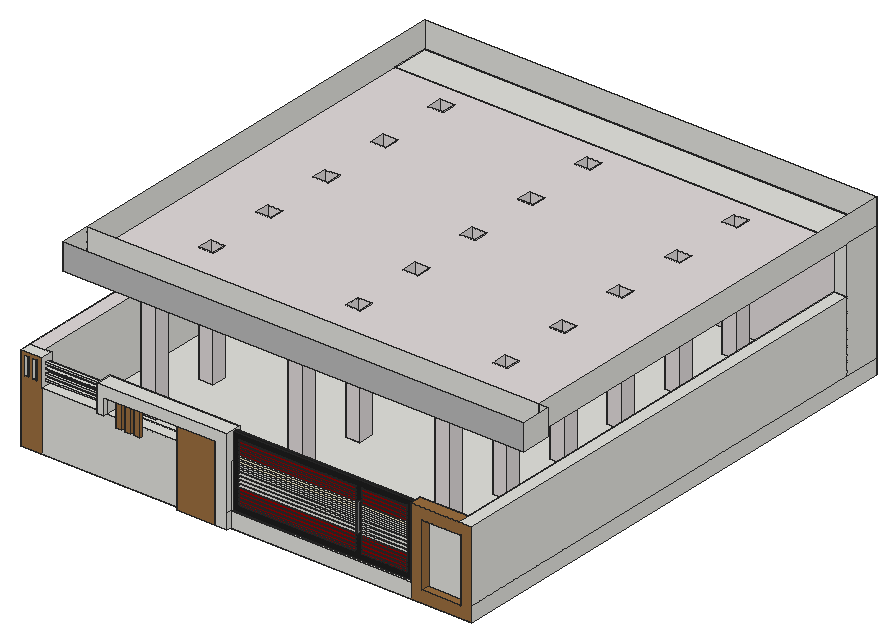
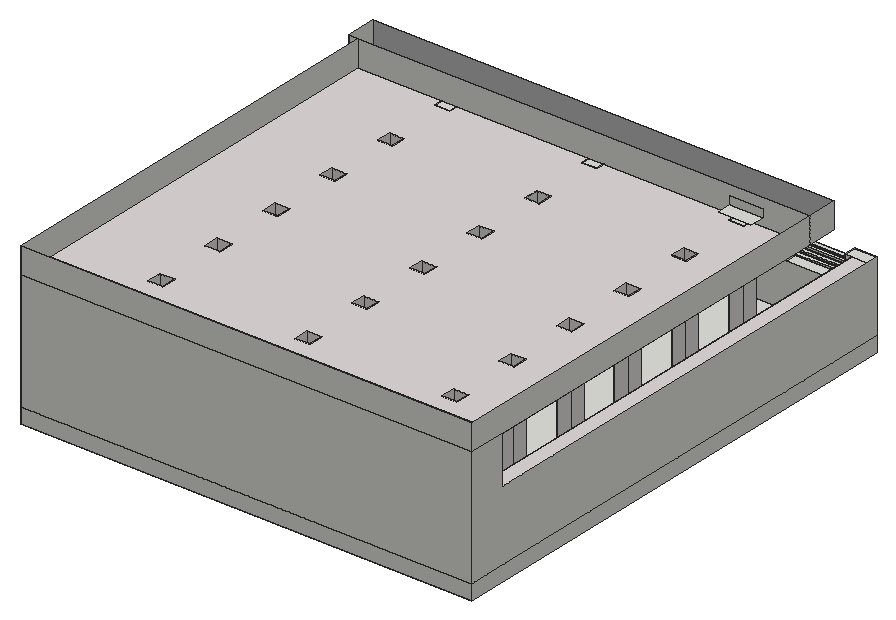
# SketchUp Ruby script. Lengths in inches.
U = 1.inch
M = Sketchup.active_model
def pt(a) = Geom::Point3d.new(a.map { |v| v * U })
def face(e, loops, mat)
  f = e.add_face(loops[0].map { |a| pt(a) })
  loops[1..].each { |l| e.add_face(l.map { |a| pt(a) }).erase! }
  f.material = f.back_material = mat if mat
  f
end
# faces: each face lists its corners as indices into pts; further lists are holes
def faces(e, pts, list, mat = nil) = list.each { |f| face(e, (f[0].is_a?(Array) ? f : [f]).map { |l| l.map { |i| pts[i] } }, mat) }
# xy, xz, yz: faces in a plane at the given z, y or x. An outline is a flat list of corners, or four numbers for a rectangle; further outlines are holes
def ring(l) = l.size == 4 ? [[l[0], l[1]], [l[2], l[1]], [l[2], l[3]], [l[0], l[3]]] : l.each_slice(2).to_a
def flat(e, list, mat, &to3) = list.each { |f| face(e, (f[0].is_a?(Array) ? f : [f]).map { |l| ring(l).map { |u, v| to3.(u, v) } }, mat) }
def xy(e, z, list, mat = nil) = flat(e, list, mat) { |x, y| [x, y, z] }
def xz(e, y, list, mat = nil) = flat(e, list, mat) { |x, z| [x, y, z] }
def yz(e, x, list, mat = nil) = flat(e, list, mat) { |y, z| [x, y, z] }
def lines(e, pts, list) = list.each { |a, b| e.add_line(pt(pts[a]), pt(pts[b])) }
# prism: a flat outline (further loops are holes) pulled along v
def prism(e, loops, v, mat = nil)
  f = face(e, loops, mat); d = Geom::Vector3d.new(v.map { |x| x * U })
  f.pushpull(f.normal.samedirection?(d) ? d.length : -d.length)
end
def box(e, o, s, mat = nil) = prism(e, [[o, [o[0] + s[0], o[1], o[2]], [o[0] + s[0], o[1] + s[1], o[2]], [o[0], o[1] + s[1], o[2]]]], [0, 0, s[2]], mat)
def at(x, y, z, deg = 0) = Geom::Transformation.translation(pt([x, y, z])) * Geom::Transformation.rotation(ORIGIN, Z_AXIS, deg.degrees)
def axes(o, x, y, z) = Geom::Transformation.new([*x, 0, *y, 0, *z, 0, *pt(o).to_a, 1])
def part(name) = M.definitions.add(name)
# library, detail: a bought-in or finely detailed component or shape, given as its bounding box
def library(name, o, s) = part(name).tap { |d| box(d.entities, o, s) }
def detail(e, o, s) = box(e.add_group.entities, o, s)
def put(e, d, t, mat = nil) = e.add_instance(d, t).tap { |i| i.material = mat if mat }
def group(e, t, mat = nil) = e.add_group.tap { |g| g.transformation = t; g.material = mat if mat }.entities
root = M.entities
M.materials.add("Generic").color = [155, 110, 63]
M.materials.add("Generic\#2").color = [186, 186, 186]
M.materials.add("Generic\#3").color = [224, 218, 218]
M.materials.add("[Color A07]").color = [153, 0, 0]
M.materials.add("[Color D01]").color = [255, 242, 204]
M.materials.add("[Color M04]").color = [142, 142, 142]
M.materials.add("[Color M08]").color = [30, 30, 30]
c1 = part("Group\#1")
xy(c1.entities,0,[[0,0,46.77,20.375]])
xz(c1.entities,0,[[0,0,46.77,11.0625]])
xy(root,-21.3125,[[275.43,0,329.375,6.375],[329.375,0,347.5625,6.375],[48.5,6.375,690.4375,724.5]])
xy(root,-5.23,[[619.21,6.375,674.35,18.4375]],"Generic")
xy(root,0.1875,[[[347.5625,6.375,603.125,6.375,603.125,23.0625,672,23.0625,672,672.375,69.875,672.375,69.875,23.0625,347.5625,23.0625],[132.71,115.57,153.71,136.82],[132.71,217.57,153.71,238.82],[132.71,319.57,153.71,340.82],[132.71,421.57,153.71,442.82],[132.71,523.57,153.71,544.82],[132.71,625.57,153.71,646.82],[341.56,625.57,362.56,646.82],[341.56,523.57,362.56,544.82],[341.56,421.57,362.56,442.82],[341.56,319.57,362.56,340.82],[341.56,217.57,362.56,238.82],[341.56,115.57,362.56,136.82],[550.4,625.57,571.4,646.82],[550.4,523.57,571.4,544.82],[550.4,421.57,571.4,442.82],[550.4,319.57,571.4,340.82],[550.4,217.57,571.4,238.82],[550.4,115.57,571.4,136.82]],[132.71,115.57,153.71,136.82],[341.56,115.57,362.56,136.82],[550.4,115.57,571.4,136.82],[132.71,217.57,153.71,238.82],
  [341.56,217.57,362.56,238.82],[550.4,217.57,571.4,238.82],[132.71,319.57,153.71,340.82],[341.56,319.57,362.56,340.82],[550.4,319.57,571.4,340.82],
  [132.71,421.57,153.71,442.82],[341.56,421.57,362.56,442.82],[550.4,421.57,571.4,442.82],[132.71,523.57,153.71,544.82],[341.56,523.57,362.56,544.82],
  [550.4,523.57,571.4,544.82],[132.71,625.57,153.71,646.82],[341.56,625.57,362.56,646.82],[550.4,625.57,571.4,646.82]])
xy(root,50.95,[[186.18,3.25,194.99,6.375],[199.43,3.25,208.24,6.375],[212.68,3.25,221.49,6.375]],"Generic")
xy(root,62.7,[[162.58,0,171.58,6.375],[79.4375,6.375,162.58,23.0625],[162.58,6.375,171.58,23.0625],[171.58,6.375,329.375,23.0625],[329.375,6.375,347.5625,23.0625]])
xy(root,69.64,[[54.75,6.375,60.37,9.625],[66.31,6.375,71.93,9.625]])
xy(root,70.21,[[79.4375,11.47,162.58,16.59],[162.58,11.47,164.83,16.59]])
xy(root,72.34,[[79.4375,11.47,162.58,16.59],[162.58,11.47,166.52,16.59]])
xy(root,77.4,[[79.4375,11.47,162.58,16.59],[162.58,11.47,166.52,16.59]])
xy(root,79.52,[[79.4375,11.47,162.58,16.59],[162.58,11.47,166.52,16.59]])
xy(root,84.59,[[79.4375,11.47,162.58,16.59],[162.58,11.47,166.52,16.59]])
xy(root,84.85,[[619.21,6.375,674.35,18.4375]],"Generic")
xy(root,85.75,[[171.58,0,275.43,6.375],[171.58,6.375,329.375,23.0625]])
xy(root,86.27,[[186.18,3.25,194.99,6.375],[199.43,3.25,208.24,6.375],[212.68,3.25,221.49,6.375]])
xy(root,86.71,[[79.4375,11.47,162.58,16.59],[162.58,11.47,166.52,16.59]])
xy(root,91.77,[[79.4375,11.47,162.58,16.59],[162.58,11.47,166.52,16.59]])
xy(root,93.9,[[79.4375,11.47,162.58,16.59],[162.58,11.47,164.83,16.59]])
xy(root,95.83,[[54.75,6.375,60.37,9.625],[66.31,6.375,71.93,9.625]])
xy(root,100.9375,[[162.58,0,347.5625,23.0625],[48.5,6.375,79.4375,23.0625],[672,6.375,690.4375,672.375]])
xy(root,100.9375,[[603.125,6.375,672,23.0625]],"Generic")
xy(root,100.9375,[[48.5,23.0625,69.875,672.375]],"Generic\#3")
xy(root,168,[[132.71,115.57,153.71,124.5],[341.56,115.57,362.56,124.5],[550.4,115.57,571.4,124.5],[132.71,124.5,153.71,136.82],[341.56,124.5,362.56,136.82],
  [550.4,124.5,571.4,136.82],[48.5,672.375,690.4375,724.5]])
xy(root,168,[[48.5,81.125,48.5,124.5,132.71,124.5,132.71,115.57,153.71,115.57,153.71,124.5,341.56,124.5,341.56,115.57,362.56,115.57,362.56,124.5,550.4,124.5,550.4,115.57,571.4,115.57,571.4,124.5,703.6875,124.5,703.6875,81.125]],"Generic\#2")
xy(root,168,[[[48.5,124.5,48.5,672.375,690.4375,672.375,690.4375,124.5,571.4,124.5,571.4,136.82,550.4,136.82,550.4,124.5,362.56,124.5,362.56,136.82,341.56,136.82,341.56,124.5,153.71,124.5,153.71,136.82,132.71,136.82,132.71,124.5],[132.71,625.57,153.71,646.82],[341.56,625.57,362.56,646.82],[550.4,625.57,571.4,646.82],[550.4,523.57,571.4,544.82],[341.56,523.57,362.56,544.82],[132.71,523.57,153.71,544.82],[341.56,421.57,362.56,442.82],[550.4,421.57,571.4,442.82],[132.71,421.57,153.71,442.82],[132.71,319.57,153.71,340.82],[341.56,319.57,362.56,340.82],[550.4,319.57,571.4,340.82],[550.4,217.57,571.4,238.82],[341.56,217.57,362.56,238.82],[132.71,217.57,153.71,238.82]]],"Generic\#3")
xz(root,0,[[329.375,-21.3125,347.5625,-21.3125,347.5625,100.9375,162.58,100.9375,162.58,62.7,171.58,62.7,171.58,85.75,329.375,85.75]])
xz(root,0,[[275.43,-21.3125,329.375,85.75]],"Generic")
xz(root,3.25,[[186.18,50.95,194.99,86.27],[199.43,50.95,208.24,86.27],[212.68,50.95,221.49,86.27]],"Generic")
xz(root,6.375,[[79.4375,-21.3125,275.43,-21.3125,275.43,62.7,221.49,62.7,221.49,50.95,212.68,50.95,212.68,62.7,208.24,62.7,208.24,50.95,199.43,50.95,199.43,62.7,194.99,62.7,194.99,50.95,186.18,50.95,186.18,62.7,79.4375,62.7],[275.43,-21.3125,329.375,62.7],[329.375,-21.3125,347.5625,62.7],[347.5625,-21.3125,603.125,0.1875],[186.18,50.95,194.99,62.7],
  [199.43,50.95,208.24,62.7],[212.68,50.95,221.49,62.7],[186.18,62.7,194.99,85.75],[199.43,62.7,208.24,85.75],[212.68,62.7,221.49,85.75],
  [275.43,62.7,329.375,85.75],[186.18,85.75,194.99,86.27],[199.43,85.75,208.24,86.27],[212.68,85.75,221.49,86.27]])
xz(root,6.375,[[[48.5,-21.3125,79.4375,100.9375],[54.75,69.64,60.37,95.83],[66.31,69.64,71.93,95.83]],[[603.125,-21.3125,690.4375,100.9375],[619.21,-5.23,674.35,84.85]]],"Generic")
xz(root,9.625,[[54.75,69.64,60.37,95.83],[66.31,69.64,71.93,95.83]])
xz(root,11.47,[[79.4375,70.21,162.58,72.34],[162.58,70.21,164.83,72.34],[164.83,72.34,166.52,77.4],[79.4375,77.4,162.58,79.52],[162.58,77.4,164.83,79.52],
  [164.83,79.52,166.52,84.59],[79.4375,84.59,162.58,86.71],[162.58,84.59,164.83,86.71],[164.83,86.71,166.52,91.77],[79.4375,91.77,162.58,93.9],
  [162.58,91.77,164.83,93.9]])
xz(root,16.59,[[79.4375,70.21,162.58,72.34],[162.58,70.21,164.83,72.34],[164.83,72.34,166.52,77.4],[79.4375,77.4,162.58,79.52],[162.58,77.4,164.83,79.52],
  [164.83,79.52,166.52,84.59],[79.4375,84.59,162.58,86.71],[162.58,84.59,164.83,86.71],[164.83,86.71,166.52,91.77],[79.4375,91.77,162.58,93.9],
  [162.58,91.77,164.83,93.9]])
xz(root,18.4375,[[619.21,-5.23,674.35,84.85]])
xz(root,23.0625,[[69.875,0.1875,347.5625,62.7],[603.125,0.1875,672,100.9375],[69.875,62.7,79.4375,100.9375],[162.58,62.7,162.58,100.9375,347.5625,100.9375,347.5625,62.7,329.375,62.7,329.375,85.75,171.58,85.75,171.58,62.7]])
xz(root,81.125,[[48.5,168,703.6875,204.9375]],"Generic\#2")
xz(root,115.57,[[132.71,0.1875,153.71,168],[341.56,0.1875,362.56,168],[550.4,0.1875,571.4,168]],"Generic\#3")
xz(root,124.5,[[48.5,168,690.4375,204.9375],[690.4375,168,703.6875,204.9375]])
xz(root,136.82,[[132.71,0.1875,153.71,168],[341.56,0.1875,362.56,168],[550.4,0.1875,571.4,168]],"Generic\#3")
xz(root,217.57,[[132.71,0.1875,153.71,168],[341.56,0.1875,362.56,168],[550.4,0.1875,571.4,168]],"Generic\#3")
xz(root,238.82,[[132.71,0.1875,153.71,168],[341.56,0.1875,362.56,168],[550.4,0.1875,571.4,168]],"Generic\#3")
xz(root,319.57,[[132.71,0.1875,153.71,168],[341.56,0.1875,362.56,168],[550.4,0.1875,571.4,168]],"Generic\#3")
xz(root,340.82,[[132.71,0.1875,153.71,168],[341.56,0.1875,362.56,168],[550.4,0.1875,571.4,168]],"Generic\#3")
xz(root,421.57,[[132.71,0.1875,153.71,168],[341.56,0.1875,362.56,168],[550.4,0.1875,571.4,168]],"Generic\#3")
xz(root,442.82,[[132.71,0.1875,153.71,168],[341.56,0.1875,362.56,168],[550.4,0.1875,571.4,168]],"Generic\#3")
xz(root,523.57,[[132.71,0.1875,153.71,168],[341.56,0.1875,362.56,168],[550.4,0.1875,571.4,168]],"Generic\#3")
xz(root,544.82,[[132.71,0.1875,153.71,168],[341.56,0.1875,362.56,168],[550.4,0.1875,571.4,168]],"Generic\#3")
xz(root,625.57,[[132.71,0.1875,153.71,168],[341.56,0.1875,362.56,168],[550.4,0.1875,571.4,168]],"Generic\#3")
xz(root,646.82,[[132.71,0.1875,153.71,168],[341.56,0.1875,362.56,168],[550.4,0.1875,571.4,168]],"Generic\#3")
xz(root,672.375,[[672,0.1875,690.4375,100.9375],[672,100.9375,690.4375,168]])
xz(root,672.375,[[69.875,0.1875,672,168],[48.5,100.9375,69.875,168]],"Generic\#3")
xz(root,724.5,[[48.5,-21.3125,690.4375,0.1875],[48.5,0.1875,690.4375,168],[48.5,168,690.4375,204.9375]])
yz(root,48.5,[[6.375,-21.3125,724.5,0.1875],[6.375,0.1875,6.375,100.9375,672.375,100.9375,672.375,168,724.5,168,724.5,0.1875],[81.125,168,124.5,204.9375],[124.5,168,724.5,204.9375]])
yz(root,54.75,[[6.375,69.64,9.625,95.83]])
yz(root,60.37,[[6.375,69.64,9.625,95.83]])
yz(root,66.31,[[6.375,69.64,9.625,95.83]])
yz(root,69.875,[[23.0625,0.1875,672.375,100.9375]])
yz(root,71.93,[[6.375,69.64,9.625,95.83]])
yz(root,79.4375,[[[6.375,62.7,23.0625,100.9375],[11.47,91.77,16.59,93.9],[11.47,84.59,16.59,86.71],[11.47,77.4,16.59,79.52],[11.47,70.21,16.59,72.34]]])
yz(root,132.71,[[115.57,0.1875,136.82,168],[217.57,0.1875,238.82,168],[319.57,0.1875,340.82,168],[421.57,0.1875,442.82,168],[523.57,0.1875,544.82,168],
  [625.57,0.1875,646.82,168]],"Generic\#3")
yz(root,153.71,[[115.57,0.1875,136.82,168],[217.57,0.1875,238.82,168],[319.57,0.1875,340.82,168],[421.57,0.1875,442.82,168],[523.57,0.1875,544.82,168],
  [625.57,0.1875,646.82,168]],"Generic\#3")
yz(root,162.58,[[[0,62.7,23.0625,100.9375],[11.47,70.21,16.59,72.34],[11.47,84.59,16.59,86.71],[11.47,77.4,16.59,79.52],[11.47,91.77,16.59,93.9]],[11.47,70.21,16.59,72.34],[11.47,77.4,16.59,79.52],[11.47,84.59,16.59,86.71],[11.47,91.77,16.59,93.9]])
yz(root,164.83,[[11.47,70.21,16.59,93.9]])
yz(root,166.52,[[11.47,72.34,16.59,77.4],[11.47,79.52,16.59,84.59],[11.47,86.71,16.59,91.77]])
yz(root,171.58,[[0,62.7,6.375,85.75],[6.375,62.7,23.0625,85.75]])
yz(root,186.18,[[3.25,50.95,6.375,86.27]],"Generic")
yz(root,194.99,[[3.25,50.95,6.375,86.27]],"Generic")
yz(root,199.43,[[3.25,50.95,6.375,86.27]],"Generic")
yz(root,208.24,[[3.25,50.95,6.375,86.27]],"Generic")
yz(root,212.68,[[3.25,50.95,6.375,86.27]],"Generic")
yz(root,221.49,[[3.25,50.95,6.375,86.27]],"Generic")
yz(root,275.43,[[0,-21.3125,6.375,85.75]],"Generic")
yz(root,329.375,[[0,-21.3125,6.375,85.75],[6.375,62.7,23.0625,85.75]])
yz(root,341.56,[[115.57,0.1875,136.82,168],[217.57,0.1875,238.82,168],[319.57,0.1875,340.82,168],[421.57,0.1875,442.82,168],[523.57,0.1875,544.82,168],
  [625.57,0.1875,646.82,168]],"Generic\#3")
yz(root,347.5625,[[0,-21.3125,6.375,0.1875],[0,0.1875,6.375,0.1875,6.375,62.7,23.0625,62.7,23.0625,100.9375,0,100.9375],[6.375,0.1875,23.0625,62.7]])
yz(root,362.56,[[115.57,0.1875,136.82,168],[217.57,0.1875,238.82,168],[319.57,0.1875,340.82,168],[421.57,0.1875,442.82,168],[523.57,0.1875,544.82,168],
  [625.57,0.1875,646.82,168]],"Generic\#3")
yz(root,550.4,[[115.57,0.1875,136.82,168],[217.57,0.1875,238.82,168],[319.57,0.1875,340.82,168],[421.57,0.1875,442.82,168],[523.57,0.1875,544.82,168],
  [625.57,0.1875,646.82,168]],"Generic\#3")
yz(root,571.4,[[115.57,0.1875,136.82,168],[217.57,0.1875,238.82,168],[319.57,0.1875,340.82,168],[421.57,0.1875,442.82,168],[523.57,0.1875,544.82,168],
  [625.57,0.1875,646.82,168]],"Generic\#3")
yz(root,603.125,[[6.375,0.1875,23.0625,100.9375]],"Generic")
yz(root,619.21,[[6.375,-5.23,18.4375,84.85]],"Generic")
yz(root,672,[[23.0625,0.1875,672.375,100.9375]])
yz(root,674.35,[[6.375,-5.23,18.4375,84.85]],"Generic")
yz(root,690.4375,[[6.375,-21.3125,724.5,0.1875],[6.375,0.1875,672.375,100.9375],[672.375,0.1875,724.5,168],[124.5,168,724.5,204.9375]])
yz(root,703.6875,[[81.125,168,124.5,204.9375]])
p = [[69.875,23.0625,0.1875],[69.875,6.375,0.1875],[162.58,13.96,70.93],[69.875,13.96,70.93],[162.58,13.96,78.18],[69.875,13.96,78.18],
  [162.58,13.96,85.43],[69.875,13.96,85.43],[162.58,13.96,92.68],[69.875,13.96,92.68]]
lines(root,p,[[0,1],[2,3],[4,5],[6,7],[8,9]])
g1 = group(root,at(347.5625,6.375,0.1875))
xy(g1,0,[[0,3.66,255.5625,8.66]],"[Color M08]")
xy(g1,10.64,[[8.11,3.66,175.29,8.66],[183.4,3.66,247.45,8.66]],"[Color A07]")
xy(g1,12.64,[[8.11,3.66,175.29,8.66],[183.4,3.66,247.45,8.66]],"[Color A07]")
xy(g1,15.64,[[8.11,3.66,175.29,8.66],[183.4,3.66,247.45,8.66]],"[Color A07]")
xy(g1,17.64,[[8.11,3.66,175.29,8.66],[183.4,3.66,247.45,8.66]],"[Color A07]")
xy(g1,20.64,[[8.11,3.66,175.29,8.66],[183.4,3.66,247.45,8.66]],"[Color A07]")
xy(g1,22.64,[[8.11,3.66,175.29,8.66],[183.4,3.66,247.45,8.66]],"[Color A07]")
xy(g1,25.64,[[8.11,3.66,175.29,8.66],[183.4,3.66,247.45,8.66]],"[Color A07]")
xy(g1,27.64,[[8.11,3.66,175.29,8.66],[183.4,3.66,247.45,8.66]],"[Color A07]")
xy(g1,30.64,[[8.11,3.66,175.29,8.66],[183.4,3.66,247.45,8.66]],"[Color A07]")
xy(g1,32.64,[[8.11,3.66,175.29,8.66],[183.4,3.66,247.45,8.66]])
xy(g1,35.04,[[178.11,0,180.64,3.66]])
xy(g1,35.64,[[8.11,3.66,175.29,8.66],[183.4,3.66,247.45,8.66]])
xy(g1,36.41,[[178.11,1.375,180.64,3.66]],"[Color M04]")
xy(g1,37.64,[[8.11,3.66,175.29,8.66],[183.4,3.66,247.45,8.66]])
xy(g1,40.64,[[8.11,3.66,175.29,8.66],[183.4,3.66,247.45,8.66]])
xy(g1,42.64,[[8.11,3.66,175.29,8.66],[183.4,3.66,247.45,8.66]])
xy(g1,45.64,[[8.11,3.66,175.29,8.66],[183.4,3.66,247.45,8.66]])
xy(g1,47.64,[[8.11,3.66,175.29,8.66],[183.4,3.66,247.45,8.66]])
xy(g1,50.64,[[8.11,3.66,175.29,8.66],[183.4,3.66,247.45,8.66]])
xy(g1,52.64,[[8.11,3.66,175.29,8.66],[183.4,3.66,247.45,8.66]])
xy(g1,55.64,[[8.11,3.66,175.29,8.66],[183.4,3.66,247.45,8.66]])
xy(g1,57.64,[[8.11,3.66,175.29,8.66],[183.4,3.66,247.45,8.66]])
xy(g1,60.64,[[8.11,3.66,175.29,8.66],[183.4,3.66,247.45,8.66]])
xy(g1,62.64,[[8.11,3.66,175.29,8.66],[183.4,3.66,247.45,8.66]])
xy(g1,65.64,[[8.11,3.66,175.29,8.66],[183.4,3.66,247.45,8.66]])
xy(g1,67.64,[[8.11,3.66,175.29,8.66],[183.4,3.66,247.45,8.66]])
xy(g1,70.64,[[8.11,3.66,175.29,8.66],[183.4,3.66,247.45,8.66]])
xy(g1,72.64,[[8.11,3.66,175.29,8.66],[183.4,3.66,247.45,8.66]],"[Color A07]")
xy(g1,73.21,[[178.11,1.375,180.64,3.66]],"[Color M04]")
xy(g1,74.59,[[178.11,0,180.64,3.66]])
xy(g1,75.64,[[8.11,3.66,175.29,8.66],[183.4,3.66,247.45,8.66]],"[Color A07]")
xy(g1,77.64,[[8.11,3.66,175.29,8.66],[183.4,3.66,247.45,8.66]],"[Color A07]")
xy(g1,80.64,[[8.11,3.66,175.29,8.66],[183.4,3.66,247.45,8.66]],"[Color A07]")
xy(g1,82.64,[[8.11,3.66,175.29,8.66],[183.4,3.66,247.45,8.66]],"[Color A07]")
xy(g1,85.64,[[8.11,3.66,175.29,8.66],[183.4,3.66,247.45,8.66]],"[Color A07]")
xy(g1,87.64,[[8.11,3.66,175.29,8.66],[183.4,3.66,247.45,8.66]],"[Color A07]")
xy(g1,90.64,[[8.11,3.66,175.29,8.66],[183.4,3.66,247.45,8.66]],"[Color A07]")
xy(g1,92.64,[[8.11,3.66,175.29,8.66],[183.4,3.66,247.45,8.66]])
xy(g1,100.75,[[0,3.66,255.5625,8.66]],"[Color M08]")
xz(g1,0,[[178.11,35.04,180.64,74.59]],"[Color M04]")
xz(g1,1.375,[[178.11,36.41,180.64,73.21]])
xz(g1,3.66,[[8.11,32.64,175.29,35.64],[183.4,32.64,247.45,35.64],[8.11,37.64,175.29,40.64],[183.4,37.64,247.45,40.64],[8.11,42.64,175.29,45.64],
  [183.4,42.64,247.45,45.64],[8.11,47.64,175.29,50.64],[183.4,47.64,247.45,50.64],[8.11,52.64,175.29,55.64],[183.4,52.64,247.45,55.64],
  [8.11,57.64,175.29,60.64],[183.4,57.64,247.45,60.64],[183.4,62.64,247.45,65.64],[178.11,73.21,180.64,74.59]])
xz(g1,3.66,[[8.11,8.11,175.29,10.64],[183.4,8.11,247.45,10.64],[8.11,12.64,175.29,15.64],[183.4,12.64,247.45,15.64],[8.11,17.64,175.29,20.64],
  [183.4,17.64,247.45,20.64],[8.11,22.64,175.29,25.64],[183.4,22.64,247.45,25.64],[8.11,27.64,175.29,30.64],[183.4,27.64,247.45,30.64],
  [8.11,72.64,175.29,75.64],[183.4,72.64,247.45,75.64],[8.11,77.64,175.29,80.64],[183.4,77.64,247.45,80.64],[8.11,82.64,175.29,85.64],
  [183.4,82.64,247.45,85.64],[8.11,87.64,175.29,90.64],[183.4,87.64,247.45,90.64]],"[Color A07]")
xz(g1,3.66,[[8.11,62.64,175.29,65.64],[8.11,67.64,175.29,70.64],[183.4,67.64,247.45,70.64]],"[Color D01]")
xz(g1,3.66,[[[0,0,255.5625,100.75],[8.11,8.11,175.29,92.64],[183.4,8.11,247.45,92.64],[178.11,73.21,180.64,74.59],[178.11,35.04,180.64,36.41]]],"[Color M08]")
xz(g1,8.66,[[[0,0,255.5625,100.75],[8.11,90.64,175.29,92.64],[8.11,85.64,175.29,87.64],[8.11,80.64,175.29,82.64],[8.11,75.64,175.29,77.64],[8.11,70.64,175.29,72.64],[8.11,65.64,175.29,67.64],[8.11,60.64,175.29,62.64],[8.11,55.64,175.29,57.64],[8.11,50.64,175.29,52.64],[8.11,45.64,175.29,47.64],[8.11,40.64,175.29,42.64],[8.11,35.64,175.29,37.64],[8.11,30.64,175.29,32.64],[8.11,25.64,175.29,27.64],[8.11,20.64,175.29,22.64],[8.11,15.64,175.29,17.64],[8.11,10.64,175.29,12.64],[183.4,10.64,247.45,12.64],[183.4,15.64,247.45,17.64],[183.4,20.64,247.45,22.64],[183.4,25.64,247.45,27.64],[183.4,30.64,247.45,32.64],[183.4,35.64,247.45,37.64],[183.4,40.64,247.45,42.64],[183.4,45.64,247.45,47.64],[183.4,50.64,247.45,52.64],[183.4,55.64,247.45,57.64],[183.4,60.64,247.45,62.64],[183.4,65.64,247.45,67.64],[183.4,70.64,247.45,72.64],[183.4,75.64,247.45,77.64],[183.4,80.64,247.45,82.64],[183.4,85.64,247.45,87.64],[183.4,90.64,247.45,92.64]]],"[Color M08]")
yz(g1,0,[[3.66,0,8.66,100.75]],"[Color M08]")
yz(g1,8.11,[[3.66,10.64,8.66,12.64],[3.66,15.64,8.66,17.64],[3.66,20.64,8.66,22.64],[3.66,25.64,8.66,27.64],[3.66,30.64,8.66,32.64],
  [3.66,35.64,8.66,37.64],[3.66,40.64,8.66,42.64],[3.66,45.64,8.66,47.64],[3.66,50.64,8.66,52.64],[3.66,55.64,8.66,57.64],
  [3.66,60.64,8.66,62.64],[3.66,65.64,8.66,67.64],[3.66,70.64,8.66,72.64],[3.66,75.64,8.66,77.64],[3.66,80.64,8.66,82.64],
  [3.66,85.64,8.66,87.64],[3.66,90.64,8.66,92.64]])
yz(g1,175.29,[[3.66,10.64,8.66,12.64],[3.66,15.64,8.66,17.64],[3.66,20.64,8.66,22.64],[3.66,25.64,8.66,27.64],[3.66,30.64,8.66,32.64],
  [3.66,35.64,8.66,37.64],[3.66,40.64,8.66,42.64],[3.66,45.64,8.66,47.64],[3.66,50.64,8.66,52.64],[3.66,55.64,8.66,57.64],
  [3.66,60.64,8.66,62.64],[3.66,65.64,8.66,67.64],[3.66,70.64,8.66,72.64],[3.66,75.64,8.66,77.64],[3.66,80.64,8.66,82.64],
  [3.66,85.64,8.66,87.64],[3.66,90.64,8.66,92.64]])
yz(g1,178.11,[[0,35.04,0,74.59,3.66,74.59,3.66,73.21,1.375,73.21,1.375,36.41,3.66,36.41,3.66,35.04]],"[Color M04]")
yz(g1,180.64,[[0,35.04,3.66,35.04,3.66,36.41,1.375,36.41,1.375,73.21,3.66,73.21,3.66,74.59,0,74.59]],"[Color M04]")
yz(g1,183.4,[[3.66,10.64,8.66,12.64],[3.66,15.64,8.66,17.64],[3.66,20.64,8.66,22.64],[3.66,25.64,8.66,27.64],[3.66,30.64,8.66,32.64],
  [3.66,35.64,8.66,37.64],[3.66,40.64,8.66,42.64],[3.66,45.64,8.66,47.64],[3.66,50.64,8.66,52.64],[3.66,55.64,8.66,57.64],
  [3.66,60.64,8.66,62.64],[3.66,65.64,8.66,67.64],[3.66,70.64,8.66,72.64],[3.66,75.64,8.66,77.64],[3.66,80.64,8.66,82.64],
  [3.66,85.64,8.66,87.64],[3.66,90.64,8.66,92.64]])
yz(g1,247.45,[[3.66,10.64,8.66,12.64],[3.66,15.64,8.66,17.64],[3.66,20.64,8.66,22.64],[3.66,25.64,8.66,27.64],[3.66,30.64,8.66,32.64],
  [3.66,35.64,8.66,37.64],[3.66,40.64,8.66,42.64],[3.66,45.64,8.66,47.64],[3.66,50.64,8.66,52.64],[3.66,55.64,8.66,57.64],
  [3.66,60.64,8.66,62.64],[3.66,65.64,8.66,67.64],[3.66,70.64,8.66,72.64],[3.66,75.64,8.66,77.64],[3.66,80.64,8.66,82.64],
  [3.66,85.64,8.66,87.64],[3.66,90.64,8.66,92.64]])
yz(g1,255.5625,[[3.66,0,8.66,100.75]],"[Color M08]")
p = [[179.12,0.6,35.64],[179.12,3.66,35.64],[179.12,3.66,73.98],[179.12,0.6,73.98]]
lines(g1,p,[[0,1],[2,3],[3,0]])
put(root,c1,at(110.7,130.3125,183.5))
